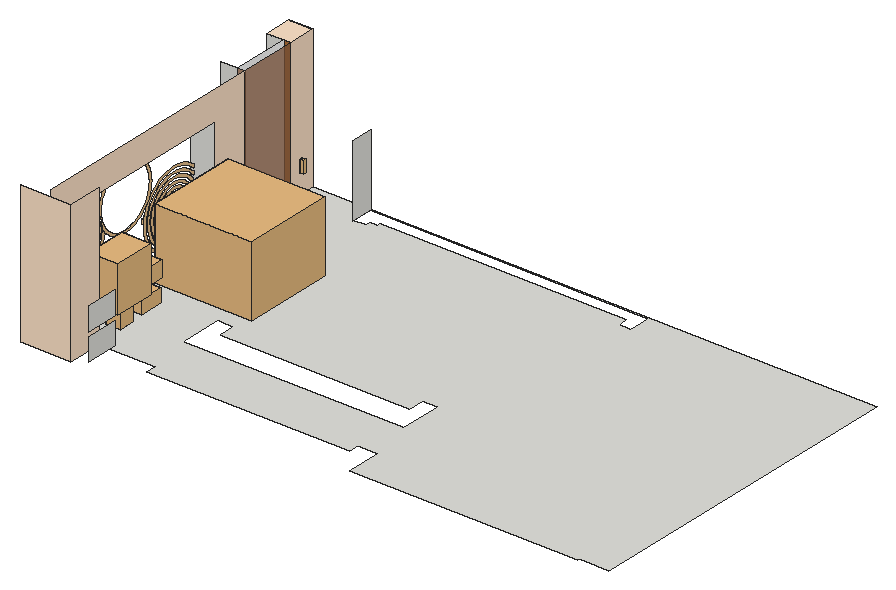
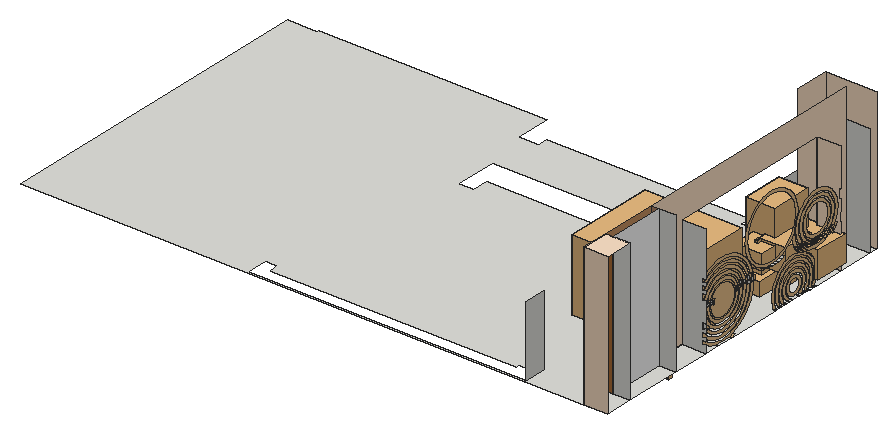
# SketchUp Ruby script. Lengths in inches.
U = 1.inch
M = Sketchup.active_model
def pt(a) = Geom::Point3d.new(a.map { |v| v * U })
def face(e, loops, mat)
  f = e.add_face(loops[0].map { |a| pt(a) })
  loops[1..].each { |l| e.add_face(l.map { |a| pt(a) }).erase! }
  f.material = f.back_material = mat if mat
  f
end
# faces: each face lists its corners as indices into pts; further lists are holes
def faces(e, pts, list, mat = nil) = list.each { |f| face(e, (f[0].is_a?(Array) ? f : [f]).map { |l| l.map { |i| pts[i] } }, mat) }
# xy, xz, yz: faces in a plane at the given z, y or x. An outline is a flat list of corners, or four numbers for a rectangle; further outlines are holes
def ring(l) = l.size == 4 ? [[l[0], l[1]], [l[2], l[1]], [l[2], l[3]], [l[0], l[3]]] : l.each_slice(2).to_a
def flat(e, list, mat, &to3) = list.each { |f| face(e, (f[0].is_a?(Array) ? f : [f]).map { |l| ring(l).map { |u, v| to3.(u, v) } }, mat) }
def xy(e, z, list, mat = nil) = flat(e, list, mat) { |x, y| [x, y, z] }
def xz(e, y, list, mat = nil) = flat(e, list, mat) { |x, z| [x, y, z] }
def yz(e, x, list, mat = nil) = flat(e, list, mat) { |y, z| [x, y, z] }
def lines(e, pts, list) = list.each { |a, b| e.add_line(pt(pts[a]), pt(pts[b])) }
# prism: a flat outline (further loops are holes) pulled along v
def prism(e, loops, v, mat = nil)
  f = face(e, loops, mat); d = Geom::Vector3d.new(v.map { |x| x * U })
  f.pushpull(f.normal.samedirection?(d) ? d.length : -d.length)
end
def box(e, o, s, mat = nil) = prism(e, [[o, [o[0] + s[0], o[1], o[2]], [o[0] + s[0], o[1] + s[1], o[2]], [o[0], o[1] + s[1], o[2]]]], [0, 0, s[2]], mat)
def at(x, y, z, deg = 0) = Geom::Transformation.translation(pt([x, y, z])) * Geom::Transformation.rotation(ORIGIN, Z_AXIS, deg.degrees)
def axes(o, x, y, z) = Geom::Transformation.new([*x, 0, *y, 0, *z, 0, *pt(o).to_a, 1])
def part(name) = M.definitions.add(name)
# library, detail: a bought-in or finely detailed component or shape, given as its bounding box
def library(name, o, s) = part(name).tap { |d| box(d.entities, o, s) }
def detail(e, o, s) = box(e.add_group.entities, o, s)
def put(e, d, t, mat = nil) = e.add_instance(d, t).tap { |i| i.material = mat if mat }
def group(e, t, mat = nil) = e.add_group.tap { |g| g.transformation = t; g.material = mat if mat }.entities
root = M.entities
M.materials.add("Material__1").color = [95, 70, 46]
M.materials.add("Material__2").color = [150, 168, 104]
M.materials.add("Material__3").color = [234, 233, 231]
M.materials.add("Material__4").color = [36, 36, 36]
M.materials.add("Material__5").color = [151, 172, 33]
M.materials.add("Material__6").color = [79, 108, 5]
M.materials.add("[Color C02]").color = [255, 228, 201]
M.materials.add("[Color M00]").color = [255, 255, 255]
M.materials.add("[Wood Bamboo]").color = [177, 112, 56]
M.materials.add("[Wood Cherry Original]").color = [152, 102, 69]
M.materials["[Wood Cherry Original]"].alpha = 0.74
M.materials.add("images").color = [235, 194, 141]
M.materials.add("wire_1").color = [140, 184, 58]
M.materials.add("wire_2").color = [244, 244, 244]
M.materials.add("wire_4").color = [86, 225, 198]
M.materials.add("wire_5").color = [232, 232, 232]
c1 = library("[SKP_VZ_MOD_01]_WALL_LIGHT",[-1.1,-1.22,0],[3.54,2.36,6.3])
c2 = library("Group\#301",[-915.9375,-34.5,735.6],[41.04,40.85,6.81])
c3 = library("Group\#300",[-991.92,-34.05,729.49],[10.64,7.28,57.53])
c4 = library("Group\#299",[-1022.2,-71.69,736.68],[86.94,78.77,45.64])
c5 = library("Group\#298",[-877.77,-100.41,669.81],[37.9,37.9,42.75])
c6 = library("Group\#297",[-957.79,-83.08,701.98],[44.29,44.29,27.78])
c7 = library("Group\#296",[-1023.9,-65.47,669.625],[67.53,67.55,39.17])
c8 = library("Group\#295",[-997.48,-49.45,708.79],[29.81,29.81,30.61])
c9 = library("Group\#294",[-956738.95,-82059.81,669752.625],[42194.58,42232.57,49521.48])
c10 = library("Group\#293",[-917.52,-36.6875,711.84],[44.99,44.98,28.22])
c11 = library("Group\#292",[-916244.63,-35413.97,669800.48],[42442.38,42642.99,59706.29])
c12 = library("Group\#291",[-955.48,-54.29,730.4],[118.63,83.7,130.4])
c13 = library("Group\#290",[-899.97,-18.72,732.17],[8.78,8.27,28.64])
c14 = library("Group\#289",[-906.16,-138.28,686.8],[98.25,106.18,75.79])
c15 = library("Group\#288",[-978.71,-103.24,719.12],[90.2,76.4,68.29])
c16 = library("Group\#287",[-955.98,-81.17,725.57],[41.03,40.85,6.81])
c17 = library("Group\#286",[-996.8,-48.73,736.67],[28.51,28.38,4.73])
c18 = library("Group\#285",[-876.58,-99.29,706.19],[35.74,35.58,5.93])
c19 = library("Group\#284",[-912.1,-32.49,735.82],[33.14,36.63,9.55])
c20 = library("Group\#283",[-994.36,-46.95,735.88],[24.38,25.9,6.88])
c21 = part("PLANT-30")
p = [[0,0,0],[1,0,0],[1,1,0]]
lines(c21.entities,p,[[0,1],[1,2],[2,0]])
put(c21.entities,c2,at(895.63,-7.06,-669.82),"Material__1")
put(c21.entities,c3,at(895.63,-7.06,-669.82),"wire_1")
put(c21.entities,c4,at(895.63,-7.06,-669.82),"Material__2")
put(c21.entities,c5,at(895.63,-7.06,-669.82),"wire_2")
put(c21.entities,c6,at(895.63,-7.06,-669.82),"wire_2")
put(c21.entities,c7,at(895.63,-7.06,-669.82),"Material__3")
put(c21.entities,c8,at(895.63,-7.06,-669.82),"wire_2")
put(c21.entities,c9,axes([895.63,-7.06,-669.82],[0.001,0,0],[0,0.001,0],[0,0,0.001]),"Material__4")
put(c21.entities,c10,at(895.63,-7.06,-669.82),"wire_2")
put(c21.entities,c11,axes([895.63,-7.06,-669.82],[0.001,0,0],[0,0.001,0],[0,0,0.001]),"Material__4")
put(c21.entities,c12,at(895.63,-7.06,-669.82),"Material__5")
put(c21.entities,c13,at(895.63,-7.06,-669.82),"wire_4")
put(c21.entities,c14,at(895.63,-7.06,-669.82),"Material__6")
put(c21.entities,c15,at(895.63,-7.06,-669.82),"Material__4")
put(c21.entities,c16,at(895.63,-7.06,-669.82),"Material__1")
put(c21.entities,c17,at(895.63,-7.06,-669.82),"Material__1")
put(c21.entities,c18,at(895.63,-7.06,-669.82),"Material__1")
put(c21.entities,c19,at(895.63,-7.06,-669.82),"wire_5")
put(c21.entities,c20,at(895.63,-7.06,-669.82),"wire_5")
c22 = library("Group\#71",[0,0,0],[82.62,78.29,61.04])
xy(root,0,[[[183.82,9,227.2,9,227.2,38.75,275.2,38.75,275.2,30,448.07,30,448.07,38.75,464.82,38.75,464.82,9,659.13,9,659.13,11,684.57,11,684.57,295.72,204.2,295.72,204.2,191.0625,183.82,191.0625,183.82,177.71,185.82,177.71,185.82,163.08,183.82,163.08,183.82,116.09,185.82,116.09,185.82,113.98,183.82,113.98,183.82,111.77,185.82,111.77,185.82,109.46,183.82,109.46,183.82,107.08,185.82,107.08,185.82,104.52,183.82,104.52,183.82,101.625,185.82,101.625,185.82,97.54,183.82,97.54,183.82,91.24,185.82,91.24,185.82,87.16,183.82,87.16,183.82,84.26,185.82,84.26,185.82,81.7,183.82,81.7,183.82,79.31,185.82,79.31,185.82,77.01,183.82,77.01,183.82,74.8,185.82,74.8,185.82,72.6875,183.82,72.6875,183.82,46.5625,204.2,46.5625,204.2,16,183.82,16],[268.13,77.03,268.13,113.97,281.8,113.97,281.8,100.22,442.97,100.22,442.97,113.97,456.63,113.97,456.63,77.03],[253.81,276.18,253.81,295.25,490.99,295.25,490.99,276.18,480.22,276.18,480.22,283.81,270.96,283.81,270.96,281.06,264.58,281.06,264.58,276.18]],[183.82,16,204.2,46.5625],[183.82,87.16,185.82,91.24],[183.82,97.54,185.82,101.625],[183.82,163.08,185.82,177.71],
  [183.82,191.0625,204.2,222.875],[183.82,222.875,197.82,272],[183.82,272,204.2,295.72]])
xy(root,0,[[197.82,222.875,204.2,272]],"[Color M00]")
xy(root,35.71,[[183.82,116.6,185.82,119.85]])
xz(root,9,[[183.82,0,227.2,120]],"[Color C02]")
xz(root,16,[[183.82,0,204.2,95.0625]])
xz(root,46.5625,[[183.82,0,183.82,37.01,184.63,37.01,184.63,44.88,183.82,44.88,183.82,54.71,185.82,54.71,185.82,62.54,183.82,62.54,183.82,95.0625,204.2,95.0625,204.2,0]],"[Color C02]")
xz(root,191.0625,[[183.82,0,204.2,0,204.2,95.0625,183.82,95.0625,183.82,56.62,185.82,56.62,185.82,53.9,183.82,53.9,183.82,51.16,185.82,51.16,185.82,48.07,183.82,48.07,183.82,44.63,185.82,44.63,185.82,40.39,183.82,40.39,183.82,22.77,185.82,22.77,185.82,18.5625,183.82,18.5625,183.82,15.12,185.82,15.12,185.82,12.03,183.82,12.03,183.82,9.27,185.82,9.27,185.82,6.59,183.82,6.59],[183.82,18.5625,185.82,22.77]])
xz(root,222.875,[[183.82,0,197.82,120]])
xz(root,222.875,[[197.82,0,204.2,120]],"[Wood Cherry Original]")
xz(root,272,[[183.82,0,197.82,120]])
xz(root,272,[[197.82,0,204.2,120]],"[Wood Bamboo]")
yz(root,185.82,[[72.6875,0,74.8,0,74.07,1.68,73.35,4.09,72.91,6.57,72.76,9.08,72.91,11.59,73.35,14.07,74.07,16.48,75.06,18.79,76.32,20.96,77.82,22.98,79.55,24.81,81.48,26.43,83.58,27.81,85.82,28.9375,88.1875,29.8,90.63,30.375,93.13,30.67,95.65,30.67,98.14,30.375,100.59,29.8,102.96,28.9375,105.2,27.81,107.3,26.43,109.23,24.81,110.96,22.98,112.46,20.96,113.71,18.79,114.71,16.48,115.43,14.07,115.87,11.59,116.01,9.08,115.87,6.57,115.43,4.09,114.71,1.68,113.98,0,116.09,0,116.53,1.02,117.32,3.65,117.8,6.34,117.95,9.08,117.8,11.82,117.32,14.51,116.53,17.14,115.45,19.66,114.08,22.03,112.44,24.23,110.5625,26.22,108.46,27.98,106.17,29.49,103.72,30.72,101.15,31.65,98.48,32.29,95.76,32.61,93.02,32.61,90.3,32.29,90.15,32.25,87.63,31.65,85.06,30.72,83.42,29.9,83.11,29.67,81.36,28.67,80.32,27.98,78.22,26.22,76.34,24.23,74.7,22.03,73.33,19.66,72.25,17.14,71.46,14.51,70.98,11.82,70.82,9.08,70.98,6.34,71.46,3.65,72.25,1.02],[77.01,0,79.31,0,78.64,1.17,77.83,3.05,77.24,5.02,76.88,7.03,76.76,9.08,76.88,11.125,77.24,13.14,77.83,15.11,78.64,16.99,79.66,18.77,80.89,20.41,82.29,21.9,83.86,23.22,85.58,24.34,87.41,25.26,89.33,25.96,91.33,26.4375,93.36,26.68,95.41,26.68,97.45,26.4375,99.44,25.96,101.37,25.26,103.2,24.34,104.91,23.22,106.48,21.9,107.89,20.41,109.12,18.77,110.14,16.99,110.95,15.11,111.54,13.14,111.9,11.125,112.01,9.08,111.9,7.03,111.54,5.02,110.95,3.05,110.14,1.17,109.46,0,111.77,0,111.93,0.27,112.83,2.37,113.49,4.55,113.88,6.8,114.01,9.08,113.88,11.36,113.49,13.61,112.83,15.79,111.93,17.89,110.79,19.86,109.42,21.69,107.86,23.35,106.11,24.82,104.2,26.08,102.16,27.1,100.02,27.88,97.8,28.41,95.53,28.67,93.25,28.67,90.98,28.41,88.76,27.88,86.62,27.1,84.58,26.08,82.67,24.82,80.92,23.35,79.36,21.69,77.99,19.86,76.85,17.89,75.95,15.79,75.29,13.61,74.9,11.36,74.76,9.08,74.9,6.8,75.29,4.55,75.95,2.37,76.85,0.27],[81.7,0,84.26,0,83.95,0.32,83.01,1.59,82.21,2.97,81.59,4.42,81.13,5.9375,80.86,7.5,80.76,9.08,80.86,10.66,81.13,12.22,81.59,13.74,82.21,15.19,83.01,16.57,83.95,17.84,85.04,18.99,86.25,20.01,87.58,20.88,88.99,21.59,90.48,22.13,92.02,22.5,93.6,22.68,95.18,22.68,96.76,22.5,98.3,22.13,99.79,21.59,101.2,20.88,102.53,20.01,103.74,18.99,104.83,17.84,105.77,16.57,106.57,15.19,107.19,13.74,107.65,12.22,107.92,10.66,108.01,9.08,107.92,7.5,107.65,5.9375,107.19,4.42,106.57,2.97,105.77,1.59,104.83,0.32,104.52,0,107.08,0,107.44,0.49,108.35,2.07,109.07,3.74,109.59,5.48,109.91,7.27,110.01,9.08,109.91,10.89,109.59,12.68,109.07,14.42,108.35,16.09,107.44,17.67,106.36,19.125,105.11,20.45,103.72,21.61,102.2,22.61,100.58,23.43,98.87,24.05,97.1,24.47,95.3,24.68,93.48,24.68,91.68,24.47,89.91,24.05,88.2,23.43,86.58,22.61,85.06,21.61,83.67,20.45,82.42,19.125,81.34,17.67,80.43,16.09,79.71,14.42,79.1875,12.68,78.87,10.89,78.76,9.08,78.87,7.27,79.1875,5.48,79.71,3.74,80.43,2.07,81.34,0.49],[87.16,0,91.24,0,90.58,0.24,89.58,0.74,88.64,1.36,87.78,2.08,87.02,2.89,86.35,3.79,85.79,4.76,85.35,5.79,85.02,6.86,84.83,7.96,84.76,9.08,84.83,10.2,85.02,11.3,85.35,12.37,85.79,13.4,86.35,14.37,87.02,15.27,87.78,16.08,88.64,16.8,89.58,17.42,90.58,17.92,91.63,18.3,92.72,18.56,93.83,18.6875,94.95,18.6875,96.0625,18.56,97.15,18.3,98.2,17.92,99.2,17.42,100.14,16.8,100.99,16.08,101.76,15.27,102.43,14.37,102.99,13.4,103.43,12.37,103.76,11.3,103.95,10.2,104.01,9.08,103.95,7.96,103.76,6.86,103.43,5.79,102.99,4.76,102.43,3.79,101.76,2.89,100.99,2.08,100.14,1.36,99.2,0.74,98.2,0.24,97.54,0,101.625,0,102.37,0.625,103.3,1.61,104.1,2.69,104.78,3.86,105.3125,5.1,105.7,6.4,105.9375,7.73,106.01,9.08,105.9375,10.43,105.7,11.76,105.3125,13.06,104.78,14.3,104.1,15.47,103.3,16.55,102.37,17.54,101.33,18.4,100.2,19.15,98.99,19.75,97.72,20.22,96.41,20.53,95.07,20.69,93.71,20.69,92.37,20.53,91.06,20.22,89.79,19.75,88.58,19.15,87.45,18.4,86.41,17.54,85.48,16.55,84.68,15.47,84,14.3,83.47,13.06,83.08,11.76,82.84,10.43,82.76,9.08,82.84,7.73,83.08,6.4,83.47,5.1,84,3.86,84.68,2.69,85.48,1.61,86.41,0.625],[163.08,0,177.71,0,178.1,0.07,181.71,1.17,185.16,2.6875,188.42,4.59,191.0625,6.59,191.0625,9.27,190.14,8.39,187.31,6.26,184.25,4.47,181.01,3.05,177.63,2.01,174.15,1.38,170.61,1.15,167.08,1.34,163.59,1.93,160.19,2.93,156.93,4.31,153.86,6.0625,151.01,8.16,148.42,10.57,146.13,13.27,144.16,16.22,142.56,19.37,141.33,22.6875,140.49,26.125,140.06,29.64,140.04,33.18,140.43,36.7,141.22,40.15,142.42,43.48,143.99,46.65,145.91,49.62,148.17,52.35,150.73,54.79,153.56,56.92,156.61,58.71,159.86,60.13,163.24,61.16,166.72,61.8,170.25,62.03,173.79,61.84,177.28,61.25,180.68,60.25,183.93,58.87,187.01,57.12,189.86,55.02,191.0625,53.9,191.0625,56.62,188.1,58.8,184.82,60.66,181.35,62.14,177.73,63.2,174.01,63.83,170.24,64.03,166.48,63.78,162.77,63.11,159.16,62,155.71,60.49,152.45,58.58,149.4375,56.3125,146.71,53.71,144.3,50.81,142.25,47.64,140.57,44.26,139.31,40.71,138.46,37.03,138.04,33.28,138.0625,29.51,138.52,25.77,139.41,22.1,140.73,18.57,142.4375,15.2,144.53,12.07,146.97,9.19,149.73,6.62,152.77,4.38,156.05,2.52,159.52,1.04],
  [[93.95,1.47,94.83,1.47,95.71,1.57,96.58,1.78,97.41,2.08,98.2,2.48,98.94,2.96,99.62,3.53,100.23,4.18,100.76,4.89,101.2,5.66,101.55,6.47,101.81,7.32,101.96,8.19,102.01,9.08,101.96,9.97,101.81,10.84,101.55,11.6875,101.2,12.5,100.76,13.27,100.23,13.98,99.62,14.625,98.94,15.2,98.2,15.68,97.41,16.08,96.58,16.38,95.71,16.59,94.83,16.69,93.95,16.69,93.07,16.59,92.2,16.38,91.37,16.08,90.58,15.68,89.84,15.2,89.16,14.625,88.55,13.98,88.02,13.27,87.58,12.5,87.22,11.6875,86.97,10.84,86.82,9.97,86.76,9.08,86.82,8.19,86.97,7.32,87.22,6.47,87.58,5.66,88.02,4.89,88.55,4.18,89.16,3.53,89.84,2.96,90.58,2.48,91.37,2.08,92.2,1.78,93.07,1.57],[94.0625,3.46,93.41,3.54,92.78,3.69,92.16,3.92,91.58,4.21,91.03,4.57,90.53,4.99,90.08,5.46,89.69,5.99,89.36,6.56,89.1,7.16,88.92,7.78,88.8,8.43,88.76,9.08,88.8,9.73,88.92,10.38,89.1,11,89.36,11.6,89.69,12.17,90.08,12.7,90.53,13.17,91.03,13.59,91.58,13.95,92.16,14.24,92.78,14.47,93.41,14.62,94.0625,14.7,94.72,14.7,95.37,14.62,96,14.47,96.62,14.24,97.2,13.95,97.75,13.59,98.25,13.17,98.7,12.7,99.09,12.17,99.42,11.6,99.68,11,99.86,10.38,99.98,9.73,100.01,9.08,99.98,8.43,99.86,7.78,99.68,7.16,99.42,6.56,99.09,5.99,98.7,5.46,98.25,4.99,97.75,4.57,97.2,4.21,96.62,3.92,96,3.69,95.37,3.54,94.72,3.46]],[170.6,3.15,173.9,3.36,177.16,3.96,180.32,4.92,183.35,6.25,186.2,7.92,188.84,9.91,191.0625,12.03,191.0625,15.12,189.77,13.5625,187.55,11.4375,185.09,9.59,182.4375,8.03,179.62,6.8,176.68,5.9,173.66,5.35,170.59,5.15,167.52,5.3125,164.49,5.83,161.54,6.69,158.71,7.89,156.04,9.42,153.56,11.24,151.3125,13.33,149.32,15.68,147.62,18.24,146.22,20.97,145.15,23.86,144.43,26.84,144.05,29.9,144.03,32.97,144.37,36.03,145.0625,39.02,146.1,41.92,147.46,44.67,149.14,47.25,151.1,49.62,153.32,51.74,155.78,53.59,158.43,55.14,161.25,56.38,164.1875,57.28,167.21,57.83,170.28,58.03,173.35,57.87,176.38,57.35,179.33,56.49,182.16,55.28,184.83,53.76,187.31,51.94,189.56,49.84,191.0625,48.07,191.0625,51.16,191,51.23,188.58,53.48,185.92,55.44,183.05,57.08,180,58.37,176.83,59.3,173.57,59.85,170.27,60.03,166.97,59.8125,163.71,59.22,160.55,58.25,157.52,56.93,154.67,55.26,152.03,53.27,149.63,50.98,147.52,48.4375,145.72,45.66,144.26,42.7,143.14,39.58,142.4,36.36,142.04,33.08,142.06,29.77,142.46,26.49,143.24,23.27,144.39,20.17,145.89,17.23,147.72,14.47,149.87,11.95,152.28,9.7,154.95,7.74,157.82,6.1,160.87,4.81,164.04,3.88,167.3,3.33],[170.58,7.15,173.41,7.33,176.21,7.84,178.93,8.68,181.53,9.82,183.98,11.25,186.25,12.96,188.31,14.92,190.12,17.11,191.0625,18.5625,191.0625,22.77,189.93,20.49,188.51,18.3,186.85,16.29,184.96,14.49,182.875,12.92,180.62,11.6,178.23,10.55,175.74,9.79,173.17,9.32,170.57,9.15,167.96,9.29,165.39,9.73,162.88,10.46,160.48,11.48,158.22,12.77,156.11,14.32,154.2,16.1,152.52,18.08,151.07,20.26,149.88,22.58,148.98,25.03,148.36,27.5625,148.04,30.15,148.03,32.76,148.32,35.35,148.9,37.9,149.78,40.35,150.9375,42.69,152.36,44.88,154.02,46.89,155.91,48.69,157.99,50.26,160.25,51.58,162.64,52.63,165.13,53.39,167.7,53.86,170.3,54.03,172.91,53.89,175.48,53.45,177.98,52.72,180.39,51.7,182.65,50.41,184.76,48.86,186.66,47.08,188.35,45.09,189.8,42.92,190.98,40.6,191.0625,40.39,191.0625,44.63,189.95,46.3,188.11,48.46,186.03,50.4,183.74,52.09,181.27,53.49,178.66,54.6,175.93,55.4,173.13,55.88,170.29,56.03,167.45,55.84,164.66,55.33,161.94,54.5,159.34,53.36,156.89,51.93,154.62,50.22,152.56,48.25,150.75,46.07,149.2,43.68,147.9375,41.14,146.98,38.46,146.34,35.69,146.03,32.87,146.05,30.02,146.39,27.2,147.07,24.44,148.05,21.78,149.34,19.25,150.92,16.88,152.76,14.71,154.84,12.78,157.125,11.09,159.6,9.6875,162.21,8.58,164.9375,7.78,167.74,7.3],[[170.55,11.15,172.93,11.3,175.26,11.73,177.54,12.43,179.71,13.38,181.77,14.58,183.66,16.01,185.38,17.65,186.9,19.48,188.19,21.48,189.25,23.61,190.05,25.84,190.58,28.16,190.84,30.52,190.83,32.9,190.54,35.26,189.98,37.57,189.15,39.79,188.07,41.91,186.76,43.89,185.22,45.7,183.48,47.32,181.5625,48.73,179.5,49.91,177.3125,50.84,175.03,51.5,172.6875,51.9,170.3125,52.03,167.94,51.875,165.6,51.45,163.33,50.75,161.15,49.8,159.1,48.6,157.21,47.17,155.49,45.53,153.97,43.7,152.67,41.7,151.62,39.57,150.82,37.34,150.29,35.02,150.02,32.66,150.04,30.28,150.33,27.92,150.89,25.61,151.72,23.38,152.8,21.27,154.11,19.29,155.65,17.48,157.39,15.86,159.3,14.45,161.37,13.27,163.56,12.34,165.84,11.68,168.18,11.28],[170.54,13.15,168.4,13.26,166.29,13.625,164.23,14.23,162.26,15.0625,160.39,16.125,158.67,17.4,157.1,18.86,155.71,20.49,154.52,22.28,153.55,24.1875,152.8,26.2,152.3,28.28,152.03,30.41,152.02,32.55,152.26,34.68,152.74,36.77,153.46,38.79,154.41,40.71,155.58,42.51,156.95,44.16,158.5,45.64,160.21,46.93,162.0625,48.02,164.03,48.88,166.08,49.5,168.1875,49.89,170.33,50.03,172.47,49.91,174.58,49.55,176.64,48.95,178.61,48.11,180.47,47.05,182.2,45.78,183.77,44.32,185.16,42.6875,186.35,40.9,187.32,38.99,188.07,36.98,188.57,34.9,188.83,32.77,188.85,30.625,188.61,28.49,188.13,26.41,187.41,24.39,186.46,22.46,185.29,20.67,183.92,19.02,182.37,17.54,180.66,16.25,178.81,15.16,176.84,14.3,174.79,13.67,172.68,13.29]],[[170.53,15.15,172.4375,15.27,174.32,15.62,176.15,16.18,177.9,16.94,179.55,17.91,181.07,19.06,182.46,20.38,183.68,21.85,184.72,23.45,185.57,25.17,186.21,26.97,186.64,28.83,186.85,30.73,186.84,32.64,186.6,34.54,186.15,36.4,185.49,38.1875,184.62,39.89,183.5625,41.48,182.32,42.94,180.93,44.24,179.39,45.375,177.72,46.32,175.96,47.07,174.13,47.61,172.25,47.93,170.34,48.03,168.43,47.9,166.55,47.5625,164.72,47,162.97,46.23,161.32,45.27,159.79,44.12,158.41,42.8,157.19,41.33,156.15,39.72,155.3,38.01,154.66,36.21,154.23,34.35,154.02,32.45,154.03,30.54,154.26,28.64,154.72,26.78,155.38,24.99,156.25,23.29,157.31,21.7,158.54,20.24,159.94,18.94,161.48,17.8,163.14,16.86,164.9,16.11,166.74,15.57,168.62,15.25],[170.52,17.15,168.84,17.24,167.1875,17.52,165.58,17.99,164.03,18.65,162.57,19.48,161.22,20.47,159.99,21.62,158.9,22.9,157.97,24.3,157.21,25.79,156.63,27.37,156.23,29,156.03,30.66,156.02,32.34,156.2,34.01,156.58,35.65,157.14,37.23,157.89,38.73,158.8,40.14,159.875,41.43,161.09,42.59,162.43,43.6,163.88,44.45,165.42,45.125,167.02,45.62,168.67,45.92,170.35,46.03,172.03,45.9375,173.68,45.66,175.29,45.18,176.84,44.53,178.3,43.7,179.65,42.7,180.88,41.56,181.96,40.28,182.89,38.88,183.66,37.39,184.24,35.8125,184.64,34.18,184.84,32.51,184.85,30.83,184.67,29.17,184.29,27.53,183.72,25.95,182.98,24.44,182.07,23.04,180.99,21.74,179.78,20.58,178.4375,19.57,176.99,18.73,175.45,18.05,173.85,17.5625,172.19,17.26]],
  [170.51,19.15,171.95,19.24,173.375,19.5,174.76,19.93,176.08,20.51,177.33,21.24,178.49,22.11,179.53,23.11,180.45,24.22,181.24,25.43,181.88,26.73,182.37,28.09,182.7,29.5,182.85,30.9375,182.85,32.39,182.67,33.82,182.33,35.23,181.83,36.58,181.17,37.87,180.37,39.08,179.43,40.18,178.37,41.16,177.21,42.02,175.95,42.74,174.62,43.3,173.23,43.71,171.81,43.95,170.36,44.03,168.92,43.93,167.49,43.67,166.11,43.25,164.79,42.67,163.54,41.94,162.38,41.07,161.34,40.07,160.41,38.96,159.625,37.74,158.99,36.45,158.5,35.09,158.17,33.68,158.01,32.24,158.02,30.79,158.2,29.36,158.54,27.95,159.04,26.6,159.7,25.31,160.5,24.1,161.4375,23,162.5,22.01,163.66,21.16,164.92,20.44,166.25,19.875,167.64,19.47,169.0625,19.23],[[69.91,27.78,72.47,27.92,74.99,28.35,77.44,29.07,79.8,30.07,82.02,31.34,84.08,32.86,85.95,34.61,87.6,36.56,89.02,38.6875,90.18,40.97,91.06,43.37,91.67,45.86,91.98,48.4,91.99,50.95,91.71,53.5,91.13,55.99,90.26,58.4,89.13,60.6875,87.73,62.83,86.1,64.8,84.25,66.57,82.2,68.1,79.99,69.39,77.65,70.42,75.2,71.16,72.68,71.62,70.13,71.78,67.57,71.65,65.05,71.21,62.6,70.49,60.24,69.49,58.02,68.22,55.96,66.71,54.09,64.96,52.4375,63.01,51.02,60.88,49.86,58.6,48.98,56.2,48.375,53.71,48.0625,51.17,48.05,48.61,48.34,46.07,48.91,43.58,49.78,41.17,50.91,38.88,52.31,36.73,53.94,34.76,55.8,33,57.84,31.46,60.05,30.17,62.39,29.15,64.84,28.4,67.36,27.94],[69.92,29.78,67.6,29.93,65.3125,30.35,63.09,31.02,60.96,31.95,58.95,33.13,57.09,34.53,55.41,36.13,53.92,37.92,52.65,39.87,51.62,41.95,50.83,44.14,50.31,46.41,50.05,48.72,50.06,51.04,50.34,53.35,50.89,55.61,51.7,57.8,52.75,59.87,54.04,61.81,55.54,63.58,57.24,65.17,59.11,66.55,61.13,67.7,63.27,68.61,65.5,69.27,67.8,69.66,70.12,69.78,72.44,69.64,74.73,69.22,76.95,68.54,79.08,67.61,81.09,66.4375,82.95,65.04,84.64,63.4375,86.12,61.65,87.39,59.7,88.42,57.61,89.21,55.42,89.73,53.16,89.99,50.85,89.98,48.52,89.7,46.21,89.15,43.95,88.35,41.77,87.29,39.7,86,37.76,84.5,35.99,82.8,34.4,80.93,33.02,78.91,31.87,76.77,30.96,74.54,30.3,72.24,29.91]],[83.42,29.9,85.06,30.72,87.63,31.65,90.15,32.25,91.39,33.71,93.11,36.3,94.52,39.07,95.6,41.99,96.33,45.01,96.47,46.17,94.91,48.28,93.98,49.89,93.97,48.27,93.64,45.5,92.98,42.79,92.01,40.17,90.75,37.68,89.2,35.36,87.4,33.23,85.36,31.32],[[69.93,31.78,72.02,31.89,74.09,32.25,76.09,32.84,78.02,33.66,79.84,34.7,81.52,35.9375,83.05,37.37,84.41,38.96,85.5625,40.71,86.51,42.57,87.24,44.54,87.73,46.57,87.98,48.65,88,50.74,87.76,52.82,87.29,54.86,86.58,56.83,85.65,58.71,84.51,60.46,83.17,62.07,81.66,63.51,79.99,64.77,78.18,65.83,76.26,66.67,74.26,67.28,72.2,67.65,70.11,67.78,68.02,67.67,65.96,67.32,63.95,66.73,62.02,65.91,60.2,64.87,58.52,63.63,56.99,62.2,55.64,60.6,54.48,58.86,53.53,56.99,52.8,55.03,52.31,53,52.06,50.92,52.05,48.83,52.28,46.75,52.75,44.71,53.46,42.74,54.39,40.86,55.53,39.11,56.87,37.5,58.38,36.05,60.06,34.79,61.86,33.74,63.78,32.9,65.78,32.29,67.84,31.92],[69.94,33.78,68.08,33.9,66.25,34.23,64.47,34.78,62.77,35.52,61.16,36.46,59.68,37.58,58.33,38.86,57.14,40.29,56.125,41.85,55.3,43.52,54.67,45.27,54.25,47.08,54.04,48.93,54.05,50.79,54.28,52.64,54.72,54.45,55.36,56.19,56.2,57.85,57.23,59.4,58.4375,60.82,59.8,62.09,61.29,63.19,62.91,64.12,64.62,64.84,66.41,65.37,68.24,65.68,70.1,65.78,71.96,65.67,73.79,65.33,75.57,64.79,77.27,64.05,78.88,63.11,80.37,61.99,81.71,60.71,82.9,59.27,83.92,57.71,84.74,56.05,85.37,54.3,85.79,52.48,86,50.63,85.99,48.77,85.76,46.93,85.33,45.12,84.68,43.375,83.84,41.71,82.81,40.17,81.6,38.75,80.24,37.48,78.75,36.37,77.13,35.45,75.42,34.72,73.63,34.2,71.8,33.88]],[[116.6,35.71,119.85,35.71,123.08,36.08,126.24,36.82,129.3,37.93,132.2,39.38,134.92,41.16,137.41,43.25,139.64,45.61,141.59,48.21,143.21,51.02,144.51,54,145.44,57.11,146.01,60.31,146.2,63.55,146.02,66.8,145.46,70,144.53,73.11,143.25,76.09,141.63,78.91,139.7,81.52,137.47,83.88,134.99,85.98,132.27,87.77,129.375,89.23,126.32,90.34,123.16,91.1,119.9375,91.48,116.6875,91.48,113.46,91.11,110.3,90.37,107.24,89.26,104.34,87.81,101.62,86.03,99.13,83.94,96.9,81.58,94.95,78.98,93.33,76.17,92.04,73.1875,91.1,70.08,90.53,66.88,90.53,66.87,90.34,63.64,90.41,62.38,90.86,61.68,92.1,59.18,93.05,56.55,93.68,53.83,93.99,51.06,93.98,49.89,94.91,48.28,96.47,46.17,96.84,45.67,99.07,43.3,101.56,41.21,104.27,39.42,107.17,37.96,110.22,36.85,113.38,36.09],[119.74,37.7,116.72,37.71,113.73,38.0625,110.8,38.76,107.96,39.8,105.27,41.15,102.75,42.82,100.45,44.76,98.38,46.95,96.58,49.375,95.08,51.99,93.89,54.76,93.03,57.65,92.51,60.62,92.34,63.63,92.52,66.64,93.04,69.61,93.91,72.5,95.11,75.27,96.625,77.88,98.43,80.29,100.5,82.49,102.81,84.42,105.34,86.07,108.03,87.42,110.87,88.45,113.81,89.14,116.8,89.49,119.82,89.48,122.8125,89.13,125.75,88.43,128.58,87.39,131.27,86.03,133.79,84.375,136.1,82.43,138.16,80.23,139.96,77.8125,141.46,75.2,142.65,72.43,143.51,69.54,144.03,66.57,144.2,63.56,144.02,60.55,143.5,57.58,142.63,54.6875,141.43,51.92,139.92,49.3125,138.11,46.89,136.04,44.7,133.73,42.77,131.2,41.12,128.51,39.77,125.67,38.74,122.74,38.05]],
  [[69.95,35.78,71.58,35.87,73.18,36.14,74.74,36.6,76.24,37.24,77.66,38.05,78.97,39.01,80.16,40.125,81.21,41.37,82.11,42.72,82.85,44.17,83.41,45.7,83.8,47.28,83.99,48.9,84,50.53,83.82,52.15,83.45,53.73,82.9,55.26,82.18,56.72,81.29,58.09,80.25,59.34,79.07,60.46,77.77,61.44,76.37,62.26,74.875,62.91,73.32,63.39,71.71,63.68,70.09,63.78,68.46,63.7,66.86,63.42,65.3,62.96,63.8,62.32,62.39,61.52,61.07,60.55,59.88,59.44,58.83,58.2,57.93,56.84,57.19,55.39,56.63,53.86,56.25,52.28,56.05,50.67,56.04,49.04,56.22,47.42,56.59,45.83,57.14,44.3,57.86,42.84,58.75,41.48,59.79,40.23,60.97,39.1,62.27,38.125,63.68,37.3,65.17,36.65,66.72,36.18,68.33,35.89],[69.96,37.78,68.57,37.87,67.2,38.12,65.86,38.53,64.58,39.09,63.38,39.79,62.26,40.63,61.25,41.59,60.36,42.66,59.6,43.83,58.98,45.08,58.51,46.4,58.19,47.76,58.04,49.14,58.04,50.54,58.21,51.93,58.54,53.28,59.03,54.59,59.66,55.83,60.43,57,61.33,58.0625,62.35,59.01,63.48,59.84,64.6875,60.53,65.97,61.08,67.3125,61.47,68.6875,61.71,70.08,61.78,71.47,61.69,72.85,61.45,74.18,61.04,75.46,60.48,76.66,59.78,77.78,58.9375,78.79,57.97,79.68,56.9,80.44,55.73,81.0625,54.48,81.53,53.17,81.85,51.81,82,50.42,82,49.03,81.83,47.64,81.5,46.28,81.02,44.98,80.38,43.73,79.61,42.57,78.71,41.51,77.6875,40.55,76.57,39.72,75.35,39.03,74.07,38.49,72.73,38.09,71.35,37.86]]],"images")
yz(root,197.82,[[222.875,0,272,120]],"[Color M00]")
yz(root,204.2,[[16,0,46.5625,0,46.5625,95.0625,191.0625,95.0625,191.0625,0,222.875,0,222.875,120,16,120]],"[Color C02]")
yz(root,204.2,[[222.875,0,272,120]],"[Wood Cherry Original]")
yz(root,227.2,[[9,0,38.75,120]],"[Color C02]")
yz(root,240.38,[[11.0625,3.75,38.75,23.0625],[11.0625,26.8125,38.75,46.125]])
yz(root,253.81,[[276.18,0,295.25,60.5625]])
p = [[183.82,86.41,0.625],[183.82,87.16,0],[185.82,87.16,0],[185.82,86.41,0.625],[183.82,91.24,0],[183.82,90.58,0.24],
  [185.82,90.58,0.24],[185.82,91.24,0],[183.82,98.2,0.24],[183.82,97.54,0],[185.82,97.54,0],[185.82,98.2,0.24],
  [183.82,101.625,0],[183.82,102.37,0.625],[185.82,102.37,0.625],[185.82,101.625,0],[183.82,159.52,1.04],[183.82,163.08,0],
  [185.82,163.08,0],[185.82,159.52,1.04],[183.82,177.71,0],[183.82,178.1,0.07],[185.82,178.1,0.07],[185.82,177.71,0],
  [183.82,190.12,17.11],[183.82,191.0625,18.5625],[185.82,191.0625,18.5625],[185.82,190.12,17.11],[183.82,191.0625,22.77],[183.82,189.93,20.49],
  [185.82,189.93,20.49],[185.82,191.0625,22.77],[185.82,78.22,26.22],[184.63,78.22,26.22],[184.63,76.34,24.23],[185.82,76.34,24.23],
  [185.82,80.32,27.98],[184.63,80.32,27.98],[185.82,81.36,28.67],[184.63,81.36,28.67],[183.82,61.86,33.74],[183.82,63.78,32.9],
  [185.82,63.78,32.9],[185.82,61.86,33.74],[183.82,53.94,34.76],[183.82,55.8,33],[185.82,55.8,33],[185.82,53.94,34.76],
  [183.82,82.8,34.4],[183.82,80.93,33.02],[185.82,80.93,33.02],[185.82,82.8,34.4],[183.82,144.03,32.97],[183.82,144.37,36.03],
  [185.82,144.37,36.03],[185.82,144.03,32.97],[183.82,58.95,33.13],[183.82,57.09,34.53],[185.82,57.09,34.53],[185.82,58.95,33.13],
  [183.82,142.4,36.36],[183.82,142.04,33.08],[185.82,142.04,33.08],[185.82,142.4,36.36],[183.82,89.2,35.36],[183.82,87.4,33.23],
  [185.82,87.4,33.23],[185.82,89.2,35.36],[183.82,140.04,33.18],[183.82,140.43,36.7],[185.82,140.43,36.7],[185.82,140.04,33.18],
  [183.82,138.46,37.03],[183.82,138.04,33.28],[185.82,138.04,33.28],[185.82,138.46,37.03],[183.82,60.06,34.79],[185.82,60.06,34.79],
  [183.82,78.02,33.66],[183.82,79.84,34.7],[185.82,79.84,34.7],[185.82,78.02,33.66],[183.82,91.39,33.71],[183.82,93.11,36.3],
  [185.82,93.11,36.3],[185.82,91.39,33.71],[183.82,158.5,35.09],[183.82,158.17,33.68],[185.82,158.17,33.68],[185.82,158.5,35.09],
  [183.82,69.94,33.78],[183.82,68.08,33.9],[185.82,68.08,33.9],[185.82,69.94,33.78],[183.82,71.8,33.88],[185.82,71.8,33.88],
  [183.82,182.67,33.82],[183.82,182.33,35.23],[185.82,182.33,35.23],[185.82,182.67,33.82],[183.82,66.25,34.23],[185.82,66.25,34.23],
  [183.82,73.63,34.2],[185.82,73.63,34.2],[183.82,156.2,34.01],[183.82,156.58,35.65],[185.82,156.58,35.65],[185.82,156.2,34.01],
  [183.82,64.47,34.78],[185.82,64.47,34.78],[183.82,75.42,34.72],[185.82,75.42,34.72],[183.82,184.24,35.8125],[183.82,184.64,34.18],
  [185.82,184.64,34.18],[185.82,184.24,35.8125],[183.82,154.66,36.21],[183.82,154.23,34.35],[185.82,154.23,34.35],[185.82,154.66,36.21],
  [183.82,84.5,35.99],[185.82,84.5,35.99],[183.82,55.41,36.13],[185.82,55.41,36.13],[183.82,186.6,34.54],[183.82,186.15,36.4],
  [185.82,186.15,36.4],[185.82,186.6,34.54],[183.82,85.95,34.61],[183.82,87.6,36.56],[185.82,87.6,36.56],[185.82,85.95,34.61],
  [183.82,77.13,35.45],[185.82,77.13,35.45],[183.82,81.52,35.9375],[185.82,81.52,35.9375],[183.82,152.26,34.68],[183.82,152.74,36.77],
  [185.82,152.74,36.77],[185.82,152.26,34.68],[183.82,52.31,36.73],[185.82,52.31,36.73],[183.82,58.38,36.05],[185.82,58.38,36.05],
  [183.82,62.77,35.52],[185.82,62.77,35.52],[183.82,188.07,36.98],[183.82,188.57,34.9],[185.82,188.57,34.9],[185.82,188.07,36.98],
  [183.82,150.82,37.34],[183.82,150.29,35.02],[185.82,150.29,35.02],[185.82,150.82,37.34],[183.82,158.99,36.45],[185.82,158.99,36.45],
  [183.82,181.83,36.58],[185.82,181.83,36.58],[183.82,190.54,35.26],[183.82,189.98,37.57],[185.82,189.98,37.57],[185.82,190.54,35.26],
  [183.82,78.75,36.37],[185.82,78.75,36.37],[183.82,90.75,37.68],[185.82,90.75,37.68],[183.82,148.32,35.35],[183.82,148.9,37.9],
  [185.82,148.9,37.9],[185.82,148.32,35.35],[183.82,61.16,36.46],[185.82,61.16,36.46],[183.82,157.14,37.23],[185.82,157.14,37.23],
  [183.82,113.38,36.09],[183.82,116.6,35.71],[185.82,116.6,35.71],[185.82,113.38,36.09],[183.82,119.85,35.71],[183.82,123.08,36.08],
  [185.82,123.08,36.08],[185.82,119.85,35.71],[183.82,146.98,38.46],[183.82,146.34,35.69],[185.82,146.34,35.69],[185.82,146.98,38.46],
  [183.82,68.33,35.89],[183.82,69.95,35.78],[185.82,69.95,35.78],[185.82,68.33,35.89],[183.82,71.58,35.87],[185.82,71.58,35.87],
  [183.82,183.66,37.39],[185.82,183.66,37.39],[183.82,66.72,36.18],[185.82,66.72,36.18],[183.82,73.18,36.14],[185.82,73.18,36.14],
  [183.82,83.05,37.37],[185.82,83.05,37.37],[183.82,86,37.76],[185.82,86,37.76],[183.82,145.0625,39.02],[185.82,145.0625,39.02],
  [183.82,53.92,37.92],[185.82,53.92,37.92],[183.82,56.87,37.5],[185.82,56.87,37.5],[183.82,74.74,36.6],[185.82,74.74,36.6],
  [183.82,110.22,36.85],[185.82,110.22,36.85],[183.82,126.24,36.82],[185.82,126.24,36.82],[183.82,65.17,36.65],[185.82,65.17,36.65],
  [183.82,155.3,38.01],[185.82,155.3,38.01],[183.82,94.52,39.07],[185.82,94.52,39.07],[183.82,80.24,37.48],[185.82,80.24,37.48],
  [183.82,143.14,39.58],[185.82,143.14,39.58],[183.82,159.625,37.74],[185.82,159.625,37.74],[183.82,185.49,38.1875],[185.82,185.49,38.1875],
  [183.82,59.68,37.58],[185.82,59.68,37.58],[183.82,76.24,37.24],[185.82,76.24,37.24],[183.82,89.02,38.6875],[185.82,89.02,38.6875],
  [183.82,181.17,37.87],[185.82,181.17,37.87],[183.82,50.91,38.88],[185.82,50.91,38.88],[183.82,63.68,37.3],[185.82,63.68,37.3],
  [183.82,141.22,40.15],[185.82,141.22,40.15],[183.82,107.17,37.96],[185.82,107.17,37.96],[183.82,129.3,37.93],[185.82,129.3,37.93],
  [183.82,153.46,38.79],[185.82,153.46,38.79]]
faces(root,p,[[0,1,2,3],[4,5,6,7],[8,9,10,11],[12,13,14,15],[16,17,18,19],[24,25,26,27],[40,41,42,43],[44,45,46,47],
  [48,49,50,51],[56,57,58,59],[60,61,62,63],[64,65,66,67],[72,73,74,75],[76,40,43,77],[78,79,80,81],[82,83,84,85],
  [86,87,88,89],[90,91,92,93],[94,90,93,95],[96,97,98,99],[91,100,101,92],[102,94,95,103],[100,108,109,101],[110,102,103,111],
  [116,117,118,119],[120,48,51,121],[57,122,123,58],[124,125,126,127],[128,129,130,131],[132,110,111,133],[79,134,135,80],[140,44,47,141],
  [142,76,77,143],[108,144,145,109],[150,151,152,153],[154,86,89,155],[97,156,157,98],[158,159,160,161],[162,132,133,163],[164,64,67,165],
  [144,170,171,145],[182,183,184,185],[186,187,188,189],[187,190,191,188],[194,186,189,195],[190,196,197,191],[134,198,199,135],[200,120,121,201],
  [122,204,205,123],[206,142,143,207],[196,208,209,197],[214,194,195,215],[216,116,119,217],[83,218,219,84],[220,162,163,221],[222,60,63,223],
  [224,154,155,225],[125,226,227,126],[170,228,229,171],[208,230,231,209],[129,232,233,130],[156,234,235,157],[236,140,141,237],[238,214,215,239]],"images")
faces(root,p,[[20,21,22,23],[28,29,30,31],[32,33,34,35],[36,37,33,32],[38,39,37,36],[52,53,54,55],[68,69,70,71],[104,105,106,107],
  [112,113,114,115],[136,137,138,139],[146,147,148,149],[166,167,168,169],[105,172,173,106],[174,175,176,177],[178,179,180,181],[192,112,115,193],
  [53,202,203,54],[210,174,177,211],[179,212,213,180],[69,240,241,70],[242,210,211,243],[212,244,245,213],[137,246,247,138]])
g1 = group(root,at(183.82,272,0),"[Color C02]")
xy(g1,120,[[0,0,20.375,23.72]])
xz(g1,23.72,[[0,0,20.375,120]])
yz(g1,20.375,[[0,0,23.72,120]])
put(root,c1,axes([206.7,203.07,-21],[-1,0,0],[0,-1.15,0],[0,0,1.64]))
put(root,c1,axes([206.7,203.07,17.07],[-1,0,0],[0,-1.15,0],[0,0,1.64]))
put(root,c1,axes([206.7,38.07,17.07],[-1,0,0],[0,-1.15,0],[0,0,1.64]))
put(root,c1,axes([206.7,282.38,17.07],[-1,0,0],[0,-1.15,0],[0,0,1.64]))
put(root,c21,axes([225.5,70.14,0.06],[0,-0.3,0],[0.3,0,0],[0,0,0.3]))
put(root,c22,at(204.2,126.98,0))
